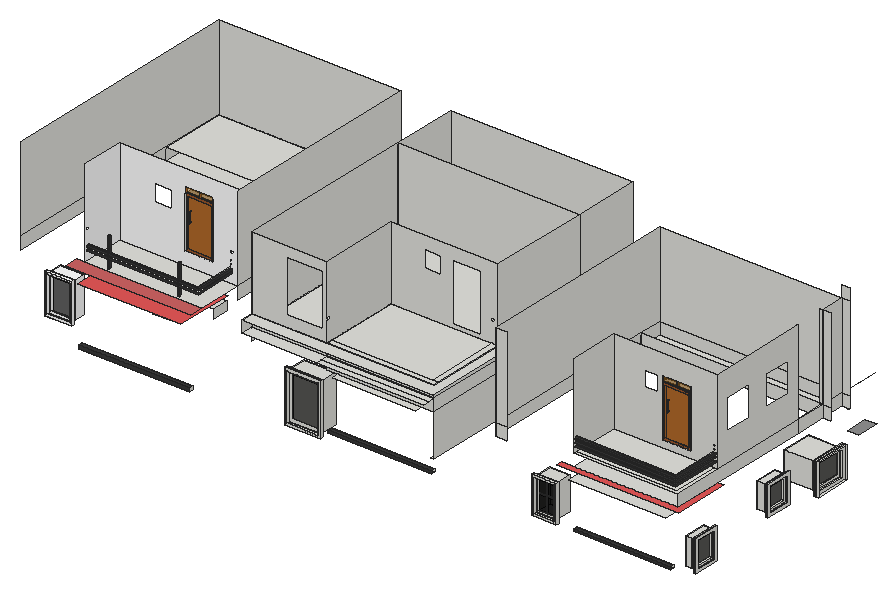
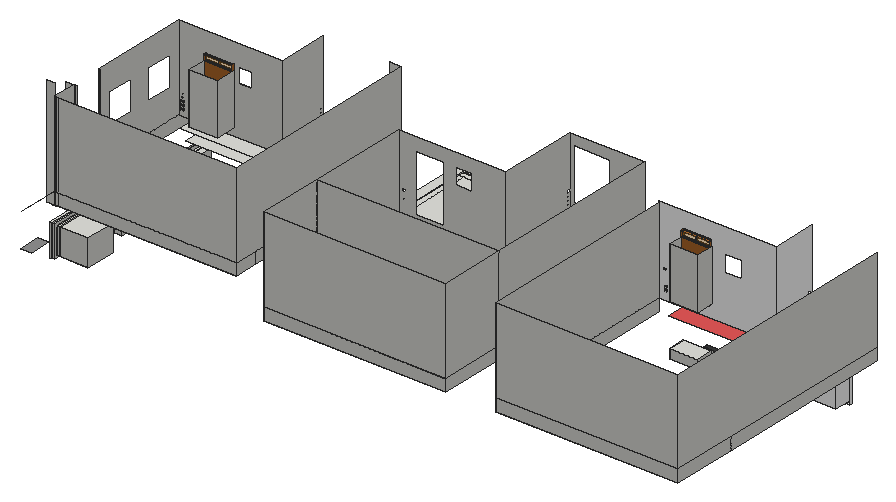
# SketchUp Ruby script. Lengths in inches.
U = 1.inch
M = Sketchup.active_model
def pt(a) = Geom::Point3d.new(a.map { |v| v * U })
def face(e, loops, mat)
  f = e.add_face(loops[0].map { |a| pt(a) })
  loops[1..].each { |l| e.add_face(l.map { |a| pt(a) }).erase! }
  f.material = f.back_material = mat if mat
  f
end
# faces: each face lists its corners as indices into pts; further lists are holes
def faces(e, pts, list, mat = nil) = list.each { |f| face(e, (f[0].is_a?(Array) ? f : [f]).map { |l| l.map { |i| pts[i] } }, mat) }
# xy, xz, yz: faces in a plane at the given z, y or x. An outline is a flat list of corners, or four numbers for a rectangle; further outlines are holes
def ring(l) = l.size == 4 ? [[l[0], l[1]], [l[2], l[1]], [l[2], l[3]], [l[0], l[3]]] : l.each_slice(2).to_a
def flat(e, list, mat, &to3) = list.each { |f| face(e, (f[0].is_a?(Array) ? f : [f]).map { |l| ring(l).map { |u, v| to3.(u, v) } }, mat) }
def xy(e, z, list, mat = nil) = flat(e, list, mat) { |x, y| [x, y, z] }
def xz(e, y, list, mat = nil) = flat(e, list, mat) { |x, z| [x, y, z] }
def yz(e, x, list, mat = nil) = flat(e, list, mat) { |y, z| [x, y, z] }
def lines(e, pts, list) = list.each { |a, b| e.add_line(pt(pts[a]), pt(pts[b])) }
# prism: a flat outline (further loops are holes) pulled along v
def prism(e, loops, v, mat = nil)
  f = face(e, loops, mat); d = Geom::Vector3d.new(v.map { |x| x * U })
  f.pushpull(f.normal.samedirection?(d) ? d.length : -d.length)
end
def box(e, o, s, mat = nil) = prism(e, [[o, [o[0] + s[0], o[1], o[2]], [o[0] + s[0], o[1] + s[1], o[2]], [o[0], o[1] + s[1], o[2]]]], [0, 0, s[2]], mat)
def at(x, y, z, deg = 0) = Geom::Transformation.translation(pt([x, y, z])) * Geom::Transformation.rotation(ORIGIN, Z_AXIS, deg.degrees)
def axes(o, x, y, z) = Geom::Transformation.new([*x, 0, *y, 0, *z, 0, *pt(o).to_a, 1])
def part(name) = M.definitions.add(name)
# library, detail: a bought-in or finely detailed component or shape, given as its bounding box
def library(name, o, s) = part(name).tap { |d| box(d.entities, o, s) }
def detail(e, o, s) = box(e.add_group.entities, o, s)
def put(e, d, t, mat = nil) = e.add_instance(d, t).tap { |i| i.material = mat if mat }
def group(e, t, mat = nil) = e.add_group.tap { |g| g.transformation = t; g.material = mat if mat }.entities
root = M.entities
M.materials.add("Generic").color = [145, 145, 145]
M.materials.add("Generic\#1").color = [206, 99, 99]
M.materials.add("Generic\#2").color = [229, 87, 87]
M.materials.add("[Color M00]").color = [255, 255, 255]
M.materials.add("[Color M07]").color = [58, 58, 58]
M.materials.add("[Color M08]").color = [45, 45, 45]
M.materials.add("[Translucent Glass Dark Green]").color = [168, 100, 12]
M.materials["[Translucent Glass Dark Green]"].alpha = 0.5
M.materials.add("[Translucent Glass Gray]").color = [0, 0, 0]
M.materials["[Translucent Glass Gray]"].alpha = 0.62
M.materials.add("[Translucent Glass Gray]1").color = [128, 128, 128]
M.materials["[Translucent Glass Gray]1"].alpha = 0.5
M.materials.add("[Wood Bamboo]").color = [177, 105, 43]
M.materials.add("[Wood Cherry Original]").color = [152, 86, 42]
c1 = part("Group\#7")
xy(c1.entities,0,[[0,0,6,43.1875]])
xy(c1.entities,3.45,[[3,3.45,6,39.74]])
xy(c1.entities,49.61,[[3,3.45,6,39.74]])
xy(c1.entities,53.0625,[[0,0,6,43.1875]])
xz(c1.entities,0,[[0,0,6,53.0625]])
xz(c1.entities,3.45,[[3,3.45,6,49.61]])
xz(c1.entities,39.74,[[3,3.45,6,49.61]])
xz(c1.entities,43.1875,[[0,0,6,53.0625]])
yz(c1.entities,0,[[0,0,43.1875,53.0625]])
yz(c1.entities,3,[[3.45,3.45,39.74,49.61]],"[Translucent Glass Gray]")
yz(c1.entities,6,[[[0,0,43.1875,53.0625],[3.45,3.45,39.74,49.61]]])
c2 = part("Group\#2")
xy(c2.entities,0,[[0,0,62.4375,3]])
xy(c2.entities,93.0625,[[0,0,62.4375,3]])
xz(c2.entities,0,[[[0,0,62.4375,93.0625],[6.31,6.31,56.13,86.75]]])
xz(c2.entities,0,[[6.31,6.31,56.13,86.75]],"[Translucent Glass Gray]")
xz(c2.entities,3,[[0,0,62.4375,93.0625]])
yz(c2.entities,0,[[0,0,3,93.0625]])
yz(c2.entities,62.4375,[[0,0,3,93.0625]])
c3 = part("Group\#6")
xy(c3.entities,0,[[0,0,6,44.5]])
xy(c3.entities,4.57,[[3,4.57,6,39.93]])
xy(c3.entities,45.43,[[3,4.57,6,39.93]])
xy(c3.entities,50,[[0,0,6,44.5]])
xz(c3.entities,0,[[0,0,6,50]])
xz(c3.entities,4.57,[[3,4.57,6,45.43]])
xz(c3.entities,39.93,[[3,4.57,6,45.43]])
xz(c3.entities,44.5,[[0,0,6,50]])
yz(c3.entities,0,[[0,0,44.5,50]])
yz(c3.entities,3,[[4.57,4.57,39.93,45.43]],"[Translucent Glass Gray]")
yz(c3.entities,6,[[[0,0,44.5,50],[4.57,4.57,39.93,45.43]]])
c4 = part("Group\#8")
xy(c4.entities,0,[[0,0,6,59.4375]])
xy(c4.entities,4.64,[[3,4.64,6,54.8]])
xy(c4.entities,46.99,[[3,4.64,6,54.8]])
xy(c4.entities,51.625,[[0,0,6,59.4375]])
xz(c4.entities,0,[[0,0,6,51.625]])
xz(c4.entities,4.64,[[3,4.64,6,46.99]])
xz(c4.entities,54.8,[[3,4.64,6,46.99]])
xz(c4.entities,59.4375,[[0,0,6,51.625]])
yz(c4.entities,0,[[0,0,59.4375,51.625]])
yz(c4.entities,3,[[4.64,4.64,54.8,46.99]],"[Translucent Glass Gray]")
yz(c4.entities,6,[[[0,0,59.4375,51.625],[4.64,4.64,54.8,46.99]]])
c5 = part("Group\#1")
xy(c5.entities,0,[[0,0,39.9375,6]])
xy(c5.entities,3.79,[[3.79,0,36.15,3]])
xy(c5.entities,60.83,[[3.79,0,36.15,3]])
xy(c5.entities,64.62,[[0,0,39.9375,6]])
xz(c5.entities,0,[[[0,0,39.9375,64.62],[3.79,3.79,36.15,60.83]]])
xz(c5.entities,3,[[18.07,3.79,20.49,3.79,20.49,32.1,36.15,32.1,36.15,34.21,20.49,34.21,20.49,60.83,18.07,60.83,18.07,34.21,3.79,34.21,3.79,32.1,18.07,32.1]],"[Color M08]")
xz(c5.entities,3,[[3.79,3.79,18.07,32.1],[20.49,3.79,36.15,32.1],[3.79,34.21,18.07,60.83],[20.49,34.21,36.15,60.83]],"[Translucent Glass Gray]")
xz(c5.entities,6,[[0,0,39.9375,64.62]],"[Translucent Glass Gray]")
yz(c5.entities,0,[[0,0,6,64.62]])
yz(c5.entities,3.79,[[0,3.79,3,60.83]])
yz(c5.entities,36.15,[[0,3.79,3,60.83]])
yz(c5.entities,39.9375,[[0,0,6,64.62]])
c6 = part("Group\#5")
xy(c6.entities,0,[[0,0,46.6875,6]],"[Color M00]")
xy(c6.entities,4.48,[[4.48,0,42.2,3]],"[Color M00]")
xy(c6.entities,67.45,[[4.48,0,42.2,3]],"[Color M00]")
xy(c6.entities,71.9375,[[0,0,46.6875,6]],"[Color M00]")
xz(c6.entities,0,[[[0,0,46.6875,71.9375],[4.48,4.48,42.2,67.45]]],"[Color M00]")
xz(c6.entities,3,[[4.48,4.48,42.2,67.45]],"[Translucent Glass Gray]")
xz(c6.entities,6,[[0,0,46.6875,71.9375]],"[Color M00]")
yz(c6.entities,0,[[0,0,6,71.9375]],"[Color M00]")
yz(c6.entities,4.48,[[0,4.48,3,67.45]],"[Color M00]")
yz(c6.entities,42.2,[[0,4.48,3,67.45]],"[Color M00]")
yz(c6.entities,46.6875,[[0,0,6,71.9375]],"[Color M00]")
c7 = part("Group\#11")
xy(c7.entities,0,[[0,0,27.8125,3]])
xy(c7.entities,27.8125,[[0,0,27.8125,3]])
xz(c7.entities,0,[[0,0,27.8125,27.8125]],"[Translucent Glass Gray]1")
xz(c7.entities,3,[[0,0,27.8125,27.8125]],"[Translucent Glass Gray]1")
yz(c7.entities,0,[[0,0,3,27.8125]])
yz(c7.entities,27.8125,[[0,0,3,27.8125]])
c8 = part("Group\#12")
xy(c8.entities,0,[[0,0,20.25,3]])
xy(c8.entities,24.8125,[[0,0,20.25,3]])
xz(c8.entities,0,[[0,0,20.25,24.8125]],"[Translucent Glass Gray]1")
xz(c8.entities,3,[[0,0,20.25,24.8125]],"[Translucent Glass Gray]1")
yz(c8.entities,0,[[0,0,3,24.8125]])
yz(c8.entities,20.25,[[0,0,3,24.8125]])
c9 = part("Group\#10")
xy(c9.entities,0,[[0,1.08,55.8125,6.01]],"[Wood Cherry Original]")
xy(c9.entities,3.96,[[3.96,1.08,51.86,3.01]],"[Wood Bamboo]")
xy(c9.entities,51.66,[[8.63,0,9.88,3.01]],"[Color M08]")
xy(c9.entities,52.54,[[8.63,0.6875,9.88,3.01]],"[Color M08]")
xy(c9.entities,71.82,[[8.63,0.6875,9.88,3.01]],"[Color M08]")
xy(c9.entities,72.69,[[8.63,0,9.88,3.01]],"[Color M08]")
xy(c9.entities,97.36,[[3.96,1.08,51.86,3.01]],"[Wood Bamboo]")
xy(c9.entities,101.3125,[[0,1.08,55.8125,6.01]],"[Wood Bamboo]")
xy(c9.entities,102.55,[[1.23,1.08,27.29,3.01],[27.29,1.08,28.52,1.95],[28.52,1.08,54.58,3.01]],"[Wood Bamboo]")
xy(c9.entities,112.31,[[1.23,1.08,1.23,3.01,27.29,3.01,27.29,1.95,28.52,1.95,28.52,3.01,54.58,3.01,54.58,1.08]],"[Wood Bamboo]")
xy(c9.entities,113.54,[[0,1.08,55.8125,6.01]],"[Wood Bamboo]")
xz(c9.entities,0,[[8.63,51.66,9.88,72.69]],"[Color M08]")
xz(c9.entities,0.6875,[[8.63,52.54,9.88,71.82]])
xz(c9.entities,1.08,[[0,101.3125,55.8125,102.55],[0,102.55,1.23,102.55,1.23,112.31,54.58,112.31,54.58,102.55,55.8125,102.55,55.8125,113.54,0,113.54]],"[Wood Bamboo]")
xz(c9.entities,1.08,[[[0,0,55.8125,101.3125],[3.96,3.96,51.86,97.36]]],"[Wood Cherry Original]")
xz(c9.entities,1.95,[[27.29,102.55,28.52,112.31]],"[Wood Bamboo]")
xz(c9.entities,3.01,[[8.63,71.82,9.88,72.69]])
xz(c9.entities,3.01,[[1.23,102.55,27.29,112.31],[28.52,102.55,54.58,112.31]],"[Translucent Glass Dark Green]")
xz(c9.entities,3.01,[[[3.96,3.96,51.86,97.36],[8.63,71.82,9.88,72.69],[8.63,51.66,9.88,52.54]]],"[Wood Bamboo]")
xz(c9.entities,6.01,[[0,0,55.8125,101.3125],[0,112.31,55.8125,113.54]],"[Wood Bamboo]")
yz(c9.entities,0,[[1.08,101.3125,6.01,113.54]],"[Wood Bamboo]")
yz(c9.entities,0,[[1.08,0,6.01,101.3125]],"[Wood Cherry Original]")
yz(c9.entities,1.23,[[1.08,102.55,3.01,112.31]],"[Wood Bamboo]")
yz(c9.entities,3.96,[[1.08,3.96,3.01,97.36]],"[Wood Bamboo]")
yz(c9.entities,8.63,[[0,51.66,0,72.69,3.01,72.69,3.01,71.82,0.6875,71.82,0.6875,52.54,3.01,52.54,3.01,51.66]],"[Color M08]")
yz(c9.entities,9.88,[[0,51.66,3.01,51.66,3.01,52.54,0.6875,52.54,0.6875,71.82,3.01,71.82,3.01,72.69,0,72.69]],"[Color M08]")
yz(c9.entities,27.29,[[1.95,102.55,3.01,112.31]],"[Wood Bamboo]")
yz(c9.entities,28.52,[[1.95,102.55,3.01,112.31]],"[Wood Bamboo]")
yz(c9.entities,51.86,[[1.08,3.96,3.01,97.36]],"[Wood Bamboo]")
yz(c9.entities,54.58,[[1.08,102.55,3.01,112.31]],"[Wood Bamboo]")
yz(c9.entities,55.8125,[[1.08,101.3125,6.01,113.54]],"[Wood Bamboo]")
yz(c9.entities,55.8125,[[1.08,0,6.01,101.3125]],"[Wood Cherry Original]")
p = [[1.23,3.01,112.31],[1.23,6.01,112.31],[9.24,3.01,71.99],[9.24,0.51,71.99],[9.24,0.51,52.37],[9.24,3.01,52.37]]
lines(c9.entities,p,[[0,1],[2,3],[3,4],[4,5]])
xy(root,813.55,[[1448.83,123.62,1452.83,175.61]])
xy(root,813.78,[[663.18,93.8125,734.35,99.8125]])
xy(root,817.95,[[1430.27,128.02,1448.83,171.21],[1448.83,128.02,1452.83,171.21]])
xy(root,818.15,[[667.55,93.8125,729.98,99.8125],[667.55,99.8125,729.98,136.8125]])
xy(root,821.06,[[330.75,76.97,332.31,80.4375],[333.5,76.97,335.06,80.4375],[330.75,80.4375,332.31,81.1],[333.5,80.4375,335.06,81.1]])
xy(root,821.06,[[[272.78,72.41,272.78,80.4375,330.75,80.4375,330.75,76.97,332.31,76.97,332.31,80.4375,333.5,80.4375,333.5,76.97,335.06,76.97,335.06,80.4375,492.5625,80.4375,492.5625,72.41],[442.43,76.97,444,79.72],[445.18,76.97,446.75,79.72]]],"[Color M07]")
xy(root,821.5625,[[1230.96,99.8125,1423.39,106.62]],"[Color M07]")
xy(root,822.31,[[741.96,103.4,947.55,111.34]],"[Color M07]")
xy(root,823.02,[[1435.83,318.51,1439.83,371.82]])
xy(root,823.79,[[1452.58,416.24,1457.58,486.33],[1457.58,416.24,1462.21,486.33]])
xy(root,824.89,[[1151.9,93.8125,1200.57,99.8125]])
xy(root,826.5,[[1230.96,99.8125,1423.39,106.62]],"[Color M07]")
xy(root,827.42,[[1414.21,322.92,1435.83,367.42],[1435.83,322.92,1439.83,367.42]])
xy(root,827.74,[[741.96,103.4,947.55,111.34]],"[Color M07]")
xy(root,828.43,[[272.78,72.41,492.5625,80.4375]],"[Color M07]")
xy(root,829.11,[[1390.02,421.57,1452.58,481],[1452.58,421.57,1457.58,481]])
xy(root,829.25,[[1156.27,93.8125,1196.2,99.8125],[1156.27,99.8125,1196.2,134.3125]])
xy(root,840.32,[[188.42,94.8125,242.3125,99.8125]],"[Color M00]")
xy(root,843.92,[[192.03,94.8125,238.71,128.125]],"[Color M00]")
xy(root,849.34,[[808.05,253.75,841.375,258.8125]])
xy(root,852.1,[[810.81,253.75,838.62,258.8125],[810.81,258.8125,838.62,292.8125]])
xy(root,852.8125,[[947.55,99.8125,954.11,258.8125]],"[Color M00]")
xy(root,855.44,[[331.98,182.0625,365.3125,187.125]])
xy(root,856.66,[[1292.01,194.1875,1317.77,199.25]])
xy(root,858.2,[[334.74,182.0625,362.55,187.125],[334.74,187.125,362.55,221.125]])
xy(root,859.42,[[1294.76,194.1875,1315.01,199.25],[1294.76,199.25,1315.01,212.4375]])
xy(root,871.01,[[1430.27,128.02,1448.83,171.21],[1448.83,128.02,1452.83,171.21]])
xy(root,875.42,[[1448.83,123.62,1452.83,175.61]])
xy(root,877.42,[[1414.21,322.92,1435.83,367.42],[1435.83,322.92,1439.83,367.42]])
xy(root,879.91,[[810.81,253.75,838.62,258.8125],[810.81,258.8125,838.62,292.8125]])
xy(root,880.74,[[1390.02,421.57,1452.58,481],[1452.58,421.57,1457.58,481]])
xy(root,881.18,[[1429.21,528.77,1451.02,572.96]],"Generic")
xy(root,881.83,[[1435.83,318.51,1439.83,371.82]])
xy(root,882.67,[[808.05,253.75,841.375,258.8125]])
xy(root,884.23,[[1294.76,194.1875,1315.01,199.25],[1294.76,199.25,1315.01,212.4375]])
xy(root,886.01,[[334.74,182.0625,362.55,187.125],[334.74,187.125,362.55,221.125]])
xy(root,886.0625,[[1452.58,416.24,1457.58,486.33],[1457.58,416.24,1462.21,486.33]])
xy(root,886.99,[[1292.01,194.1875,1317.77,199.25]])
xy(root,888.77,[[331.98,182.0625,365.3125,187.125]])
xy(root,889.29,[[862.0625,258.8125,917.875,288.3125]])
xy(root,890.49,[[1327.46,199.25,1383.27,240]])
xy(root,893.875,[[1156.27,93.8125,1196.2,99.8125],[1156.27,99.8125,1196.2,134.3125]])
xy(root,898.24,[[1151.9,93.8125,1200.57,99.8125]])
xy(root,902.05,[[392.26,187.125,448.07,220.9375]])
xy(root,911.21,[[667.55,93.8125,729.98,99.8125],[667.55,99.8125,729.98,136.8125]])
xy(root,915.58,[[663.18,93.8125,734.35,99.8125]])
xy(root,915.85,[[192.03,94.8125,238.71,128.125]],"[Color M00]")
xy(root,917.875,[[1230.96,88,1423.39,199.25]])
xy(root,919.45,[[188.42,94.8125,242.3125,99.8125]],"[Color M00]")
xy(root,936,[[764.52,86,929.22,99.8125],[741.96,99.8125,954.11,258.8125],[1230.96,99.8125,1435.83,199.25],[1409.33,398.12,1435.83,459.8125],[135.5,459.8125,495.5,590.625],
  [594.11,459.8125,954.11,590.625],[1075.83,459.8125,1409.33,507.5625],[1409.33,459.8125,1435.83,507.5625],[1075.83,507.5625,1409.33,507.75],[1409.33,507.5625,1429.21,507.75],
  [1429.21,507.5625,1435.83,507.75],[1435.83,507.5625,1451.02,507.75]])
xy(root,936,[[272.78,71.5,475.8125,187.125],[1207.39,88,1448.83,88,1448.83,199.25,1435.83,199.25,1435.83,99.8125,1207.39,99.8125]],"Generic\#2")
xy(root,960,[[594.11,74.75,741.96,99.8125],[741.96,74.75,954.11,86],[741.96,86,954.11,99.8125],[[263.03,99.8125,495.5,187.125],[444.65,105.3,446.21,109.43],[441.9,105.3,443.46,109.43],[303.36,105.3,304.92,108.8],[306.11,105.3,307.67,108.8]],[594.11,99.8125,594.11,459.8125,954.11,459.8125,954.11,258.8125,741.96,258.8125,741.96,99.8125],
  [1230.96,99.8125,1230.96,106.4375,1429.96,106.4375,1429.96,199.25,1435.83,199.25,1435.83,99.8125],[303.36,105.3,304.92,108.8],[306.11,105.3,307.67,108.8],[441.9,105.3,443.46,109.43],[444.65,105.3,446.21,109.43],
  [1230.96,106.4375,1429.96,199.25],[1433.58,398.12,1435.83,459.8125],[135.5,459.8125,495.5,590.625],[594.11,459.8125,954.11,590.625],[1433.58,459.8125,1435.83,507.5625],
  [1433.58,507.5625,1435.83,507.75]])
xy(root,960,[[248.28,71.5,495.5,99.8125]],"Generic\#1")
xy(root,970.67,[[1230.96,101.06,1230.96,106.62,1426.46,106.62,1426.46,199.25,1432.02,199.25,1432.02,101.06]],"[Color M07]")
xy(root,973.42,[[1230.96,101.06,1432.02,101.06,1432.02,199.25,1426.46,199.25,1426.46,106.62,1230.96,106.62]],"[Color M07]")
xy(root,974.55,[[1327.46,199.25,1383.27,240]])
xy(root,977.18,[[263.03,103.78,263.03,109.42,479.41,109.42,479.41,187.125,485.0625,187.125,485.0625,103.78]],"[Color M07]")
xy(root,977.8,[[1230.96,101.06,1230.96,106.62,1426.46,106.62,1426.46,199.25,1432.02,199.25,1432.02,101.06]],"[Color M07]")
xy(root,980.55,[[1230.96,101.06,1432.02,101.06,1432.02,199.25,1426.46,199.25,1426.46,106.62,1230.96,106.62]],"[Color M07]")
xy(root,980.56,[[263.03,103.78,485.0625,103.78,485.0625,187.125,479.41,187.125,479.41,109.42,263.03,109.42]])
xy(root,983.6875,[[594.11,74.75,972.24,74.75,972.24,260.5,954.11,260.5,954.11,99.8125,594.11,99.8125],[741.96,99.8125,954.11,111.125],[741.96,111.125,942.11,258.8125],[942.11,111.125,954.11,258.8125]])
xy(root,983.81,[[263.03,103.78,263.03,109.42,479.41,109.42,479.41,187.125,485.0625,187.125,485.0625,103.78]],"[Color M07]")
xy(root,984.61,[[1230.96,101.06,1230.96,106.62,1426.46,106.62,1426.46,199.25,1432.02,199.25,1432.02,101.06]],"[Color M07]")
xy(root,985.81,[[391.33,187.125,447.14,220.9375]])
xy(root,987.18,[[263.03,103.78,485.0625,103.78,485.0625,187.125,479.41,187.125,479.41,109.42,263.03,109.42]],"[Color M07]")
xy(root,987.36,[[1230.96,101.06,1432.02,101.06,1432.02,199.25,1426.46,199.25,1426.46,106.62,1230.96,106.62]],"[Color M07]")
xz(root,72.41,[[272.78,821.06,492.5625,828.43]],"[Color M07]")
xz(root,80.4375,[[272.78,821.06,492.5625,828.43]])
xz(root,93.8125,[[[663.18,813.78,734.35,915.58],[667.55,818.15,729.98,911.21]],[[1151.9,824.89,1200.57,898.24],[1156.27,829.25,1196.2,893.875]]])
xz(root,94.8125,[[[188.42,840.32,242.3125,919.45],[192.03,843.92,238.71,915.85]]],"[Color M00]")
xz(root,99.8125,[[[663.18,813.78,734.35,915.58],[667.55,818.15,729.98,911.21]],[[1151.9,824.89,1200.57,898.24],[1156.27,829.25,1196.2,893.875]],[741.96,936,954.11,960],[1075.83,936,1098.52,960],[594.11,960,741.96,983.6875],
  [741.96,960,954.11,983.6875],[1075.83,960,1098.52,1128],[[594.11,983.6875,741.96,1128],[663.18,1006.65,734.35,1108.45]]])
xz(root,99.8125,[[1230.96,821.5625,1423.39,826.5]],"[Color M07]")
xz(root,101.06,[[1230.96,970.67,1432.02,973.42],[1230.96,977.8,1432.02,980.55],[1230.96,984.61,1432.02,987.36]],"[Color M07]")
xz(root,103.4,[[741.96,822.31,947.55,827.74]],"[Color M07]")
xz(root,103.78,[[263.03,977.18,485.0625,980.56],[263.03,983.81,485.0625,987.18]],"[Color M07]")
xz(root,105.3,[[303.36,960,304.92,1017.95],[306.11,960,307.67,1017.95],[441.9,960,443.46,1017.95],[444.65,960,446.21,1017.95]],"[Color M07]")
xz(root,106.62,[[1230.96,821.5625,1423.39,826.5],[1230.96,970.67,1426.46,973.42],[1230.96,977.8,1426.46,980.55],[1230.96,984.61,1426.46,987.36]])
xz(root,108.8,[[303.36,960,304.92,1017.95],[306.11,960,307.67,1017.95]])
xz(root,109.42,[[263.03,977.18,479.41,980.56],[263.03,983.81,479.41,987.18]])
xz(root,109.43,[[441.9,960,443.46,1017.95],[444.65,960,446.21,1017.95]])
xz(root,111.34,[[741.96,822.31,947.55,827.74]])
xz(root,123.62,[[1448.83,813.55,1452.83,875.42]])
xz(root,128.02,[[1430.27,817.95,1448.83,871.01],[1448.83,817.95,1452.83,871.01]])
xz(root,128.125,[[192.03,843.92,238.71,915.85]],"[Color M00]")
xz(root,134.3125,[[1156.27,829.25,1196.2,893.875]])
xz(root,136.8125,[[667.55,818.15,729.98,911.21]])
xz(root,171.21,[[1430.27,817.95,1448.83,871.01],[1448.83,817.95,1452.83,871.01]])
xz(root,175.61,[[1448.83,813.55,1452.83,875.42]])
xz(root,182.0625,[[[331.98,855.44,365.3125,888.77],[334.74,858.2,362.55,886.01]]])
xz(root,187.125,[[[331.98,855.44,365.3125,888.77],[334.74,858.2,362.55,886.01]]])
xz(root,187.125,[[[263.03,960,495.5,1132.1875],[391.33,985.81,447.14,1101.01],[331.98,1051,365.3125,1084.33],[479.41,1013.31,487.4375,1018.25],[479.41,977.18,485.0625,980.56],[479.41,983.81,485.0625,987.18],[479.41,991.25,485.0625,994.62],[479.41,998.31,485.0625,1001.68]]],"[Color M00]")
xz(root,194.1875,[[[1292.01,856.66,1317.77,886.99],[1294.76,859.42,1315.01,884.23]]])
xz(root,199.25,[[[1292.01,856.66,1317.77,886.99],[1294.76,859.42,1315.01,884.23]],[[1230.96,960,1435.83,1128],[1327.46,974.55,1383.27,1088.1],[1292.01,1055.54,1317.77,1085.86],[1426.46,998.375,1432.02,1001.125],[1426.46,991.4375,1432.02,994.1875],[1426.46,984.61,1432.02,987.36],[1426.46,977.8,1432.02,980.55],[1426.46,970.67,1432.02,973.42]]])
xz(root,212.4375,[[1294.76,859.42,1315.01,884.23]])
xz(root,220.9375,[[392.26,884.16,448.07,902.05],[391.33,985.81,447.14,1087.12]])
xz(root,221.125,[[334.74,858.2,362.55,886.01]])
xz(root,240,[[1327.46,880.74,1383.27,890.49],[1327.46,974.55,1383.27,1075.87]])
xz(root,253.75,[[[808.05,849.34,841.375,882.67],[810.81,852.1,838.62,879.91]]])
xz(root,258.8125,[[[808.05,849.34,841.375,882.67],[810.81,852.1,838.62,879.91]],[741.96,960,954.11,983.6875],[[741.96,983.6875,954.11,1128],[863.52,990.21,919.33,1104.02],[808.05,1069.84,841.375,1103.17],[939.83,1022.6875,947.77,1028.125],[939.83,1015.6875,944.64,1017.5625],[939.83,1008.5625,944.64,1010.4375],[939.83,1001.7,944.64,1003.57],[939.83,994.52,944.64,996.39]]])
xz(root,288.3125,[[862.0625,877.58,917.875,889.29]])
xz(root,292.8125,[[810.81,852.1,838.62,879.91]])
xz(root,318.51,[[1435.83,823.02,1439.83,881.83]])
xz(root,322.92,[[1414.21,827.42,1435.83,877.42],[1435.83,827.42,1439.83,877.42]])
xz(root,367.42,[[1414.21,827.42,1435.83,877.42],[1435.83,827.42,1439.83,877.42]])
xz(root,371.82,[[1435.83,823.02,1439.83,881.83]])
xz(root,398.12,[[1433.58,960,1435.83,1128]])
xz(root,416.24,[[1452.58,823.79,1457.58,886.0625],[1457.58,823.79,1462.21,886.0625]])
xz(root,421.57,[[1390.02,829.11,1452.58,880.74],[1452.58,829.11,1457.58,880.74]])
xz(root,459.8125,[[594.11,936,954.11,960],[1075.83,936,1429.21,960],[1429.21,936,1433.58,960],[1433.58,936,1435.83,960],[1435.83,936,1451.02,960],
  [594.11,960,954.11,1128],[1429.21,960,1433.58,1128],[1433.58,960,1435.83,1128],[1435.83,960,1451.02,1128]])
xz(root,481,[[1390.02,829.11,1452.58,880.74],[1452.58,829.11,1457.58,880.74]])
xz(root,486.33,[[1452.58,823.79,1457.58,886.0625],[1457.58,823.79,1462.21,886.0625]])
xz(root,507.5625,[[1075.83,936,1429.21,960],[1429.21,936,1451.02,960],[1075.83,960,1429.21,1128],[1429.21,960,1451.02,1128]])
xz(root,507.75,[[1435.83,936,1451.02,1152],[1433.58,960,1435.83,1128]])
xz(root,590.625,[[135.5,936,495.5,960],[594.11,936,954.11,960],[135.5,960,495.5,1128],[594.11,960,954.11,1128]])
yz(root,135.5,[[99.8125,936,459.8125,960],[459.8125,936,590.625,960],[99.8125,960,590.625,1128]])
yz(root,188.42,[[94.8125,840.32,99.8125,919.45]],"[Color M00]")
yz(root,192.03,[[94.8125,843.92,128.125,915.85]],"[Color M00]")
yz(root,238.71,[[94.8125,843.92,128.125,915.85]],"[Color M00]")
yz(root,242.3125,[[94.8125,840.32,99.8125,919.45]],"[Color M00]")
yz(root,263.03,[[103.78,977.18,109.42,980.56],[103.78,983.81,109.42,987.18]])
yz(root,263.03,[[[99.8125,960,106.6,960,106.6,977.18,103.78,977.18,103.78,980.56,109.42,980.56,109.42,977.18,106.6,977.18,106.6,960,187.125,960,187.125,1132.1875,99.8125,1132.1875],[101.4,1013.31,109.42,1018.25],[103.78,983.81,109.42,987.18],[103.78,991.25,109.42,994.62],[103.78,998.31,109.42,1001.68]]],"[Color M00]")
yz(root,272.78,[[72.41,821.06,80.4375,828.43]])
yz(root,303.36,[[105.3,960,108.8,1017.95]],"[Color M07]")
yz(root,304.92,[[105.3,960,108.8,1017.95]],"[Color M07]")
yz(root,306.11,[[105.3,960,108.8,1017.95]],"[Color M07]")
yz(root,307.67,[[105.3,960,108.8,1017.95]],"[Color M07]")
yz(root,331.98,[[182.0625,855.44,187.125,888.77]])
yz(root,334.74,[[182.0625,858.2,187.125,886.01],[187.125,858.2,221.125,886.01]])
yz(root,362.55,[[182.0625,858.2,187.125,886.01],[187.125,858.2,221.125,886.01]])
yz(root,365.3125,[[182.0625,855.44,187.125,888.77]])
yz(root,391.33,[[187.125,985.81,220.9375,1087.12]])
yz(root,392.26,[[187.125,884.16,220.9375,902.05]])
yz(root,441.9,[[105.3,960,109.43,1017.95]],"[Color M07]")
yz(root,443.46,[[105.3,960,109.43,1017.95]],"[Color M07]")
yz(root,444.65,[[105.3,960,109.43,1017.95]],"[Color M07]")
yz(root,446.21,[[105.3,960,109.43,1017.95]],"[Color M07]")
yz(root,447.14,[[187.125,985.81,220.9375,1087.12]])
yz(root,448.07,[[187.125,884.16,220.9375,902.05]])
yz(root,479.41,[[109.42,977.18,187.125,980.56],[109.42,983.81,187.125,987.18]])
yz(root,485.0625,[[103.78,977.18,187.125,980.56],[103.78,983.81,187.125,987.18]],"[Color M07]")
yz(root,492.5625,[[72.41,821.06,80.4375,828.43]])
yz(root,495.5,[[187.125,936,590.625,960],[187.125,960,590.625,1128]])
yz(root,594.11,[[99.8125,936,99.8125,960,74.75,960,74.75,983.6875,99.8125,983.6875,99.8125,960,459.8125,960,459.8125,936],[459.8125,936,590.625,960],[99.8125,960,459.8125,1128],[459.8125,960,590.625,1128]])
yz(root,663.18,[[93.8125,813.78,99.8125,915.58]])
yz(root,667.55,[[93.8125,818.15,99.8125,911.21],[99.8125,818.15,136.8125,911.21]])
yz(root,729.98,[[93.8125,818.15,99.8125,911.21],[99.8125,818.15,136.8125,911.21]])
yz(root,734.35,[[93.8125,813.78,99.8125,915.58]])
yz(root,741.96,[[103.4,822.31,111.34,827.74],[99.8125,960,258.8125,983.6875],[[99.8125,983.6875,258.8125,983.6875,258.8125,1128,99.8125,1128,99.8125,1028.125,107.75,1028.125,107.75,1022.6875,99.8125,1022.6875],[102.9375,994.52,107.75,996.39],[102.9375,1001.7,107.75,1003.57],[102.9375,1008.5625,107.75,1010.4375],[102.9375,1015.6875,107.75,1017.5625]]])
yz(root,808.05,[[253.75,849.34,258.8125,882.67]])
yz(root,810.81,[[253.75,852.1,258.8125,879.91],[258.8125,852.1,292.8125,879.91]])
yz(root,838.62,[[253.75,852.1,258.8125,879.91],[258.8125,852.1,292.8125,879.91]])
yz(root,841.375,[[253.75,849.34,258.8125,882.67]])
yz(root,862.0625,[[258.8125,877.58,288.3125,889.29]])
yz(root,917.875,[[258.8125,877.58,288.3125,889.29]])
yz(root,954.11,[[99.8125,852.8125,258.8125,936],[258.8125,852.8125,260.5,936],[99.8125,936,260.5,960],[260.5,936,459.8125,960],[459.8125,936,590.625,960],
  [99.8125,960,258.8125,983.6875],[258.8125,960,260.5,983.6875],[260.5,960,459.8125,960,459.8125,1128,258.8125,1128,258.8125,983.6875,260.5,983.6875],[459.8125,960,590.625,1128]])
yz(root,1075.83,[[99.8125,936,459.8125,960],[459.8125,936,507.5625,960],[99.8125,960,507.5625,1128]])
yz(root,1151.9,[[93.8125,824.89,99.8125,898.24]])
yz(root,1156.27,[[93.8125,829.25,99.8125,893.875],[99.8125,829.25,134.3125,893.875]])
yz(root,1196.2,[[93.8125,829.25,99.8125,893.875],[99.8125,829.25,134.3125,893.875]])
yz(root,1200.57,[[93.8125,824.89,99.8125,898.24]])
yz(root,1230.96,[[99.8125,821.5625,106.62,826.5],[[99.8125,960,199.25,1128],[101.06,970.67,106.62,973.42],[101.06,977.8,106.62,980.55],[101.06,984.61,106.62,987.36],[101.06,991.4375,106.62,994.1875],[101.06,998.375,106.62,1001.125]],[101.06,970.67,106.62,973.42],[101.06,977.8,106.62,980.55],[101.06,984.61,106.62,987.36]])
yz(root,1292.01,[[194.1875,856.66,199.25,886.99]])
yz(root,1294.76,[[194.1875,859.42,199.25,884.23],[199.25,859.42,212.4375,884.23]])
yz(root,1315.01,[[194.1875,859.42,199.25,884.23],[199.25,859.42,212.4375,884.23]])
yz(root,1317.77,[[194.1875,856.66,199.25,886.99]])
yz(root,1327.46,[[199.25,880.74,240,890.49],[199.25,974.55,240,1075.87]])
yz(root,1383.27,[[199.25,880.74,240,890.49],[199.25,974.55,240,1075.87]])
yz(root,1390.02,[[421.57,829.11,481,880.74]])
yz(root,1414.21,[[322.92,827.42,367.42,877.42]])
yz(root,1426.46,[[106.62,970.67,199.25,973.42],[106.62,977.8,199.25,980.55],[106.62,984.61,199.25,987.36]])
yz(root,1430.27,[[128.02,817.95,171.21,871.01]])
yz(root,1432.02,[[101.06,970.67,199.25,973.42],[101.06,977.8,199.25,980.55],[101.06,984.61,199.25,987.36]],"[Color M07]")
yz(root,1435.83,[[[318.51,823.02,371.82,881.83],[322.92,827.42,367.42,877.42]],[99.8125,936,398.12,960],[398.12,936,459.8125,960],[459.8125,936,507.75,960],[[199.25,960,398.12,1128],[223.32,1017.77,276.63,1076.58],[318.51,1017.77,371.82,1076.58]],
  [459.8125,960,507.75,1128]])
yz(root,1439.83,[[[318.51,823.02,371.82,881.83],[322.92,827.42,367.42,877.42]]])
yz(root,1448.83,[[[123.62,813.55,175.61,875.42],[128.02,817.95,171.21,871.01]]])
yz(root,1452.58,[[[416.24,823.79,486.33,886.0625],[421.57,829.11,481,880.74]]])
yz(root,1452.83,[[[123.62,813.55,175.61,875.42],[128.02,817.95,171.21,871.01]]])
yz(root,1457.58,[[[416.24,823.79,486.33,886.0625],[421.57,829.11,481,880.74]]])
p = [[263.03,99.8125,936],[263.03,99.8125,935.375],[272.78,77.5,823],[475.8125,77.5,823],[263.03,105.8125,979],[483.03,105.8125,979],
  [483.03,187.125,979],[263.03,105.8125,986],[483.03,105.8125,986],[483.03,187.125,986],[1435.83,507.75,960],[1435.83,590.625,960],
  [741.96,108.79,823],[947.55,108.79,823],[1230.96,103.125,972],[1429.96,103.125,972],[1429.96,199.25,972],[1230.96,103.125,979],
  [1429.96,103.125,979],[1429.96,199.25,979],[1230.96,103.125,986],[1429.96,103.125,986],[1429.96,199.25,986],[1230.96,103.9375,823],
  [1423.39,103.9375,823]]
lines(root,p,[[0,1],[2,3],[4,5],[5,6],[7,8],[8,9],[10,11],[12,13],[14,15],[15,16],[17,18],[18,19],
  [20,21],[21,22],[23,24]])
put(root,c1,at(1442.83,128.02,817.95))
put(root,c2,at(667.55,99.8125,818.15))
put(root,c3,at(1429.83,322.92,827.42))
put(root,c4,at(1446.58,421.57,829.11))
put(root,c5,at(1156.27,99.8125,829.25))
put(root,c6,at(192.03,99.8125,843.92))
put(root,c7,at(810.81,258.8125,852.1))
put(root,c7,at(334.74,187.125,858.2))
put(root,c8,at(1294.76,199.25,859.42))
put(root,c9,at(1327.46,198.17,974.55))
put(root,c9,at(391.33,187.125,985.81))
